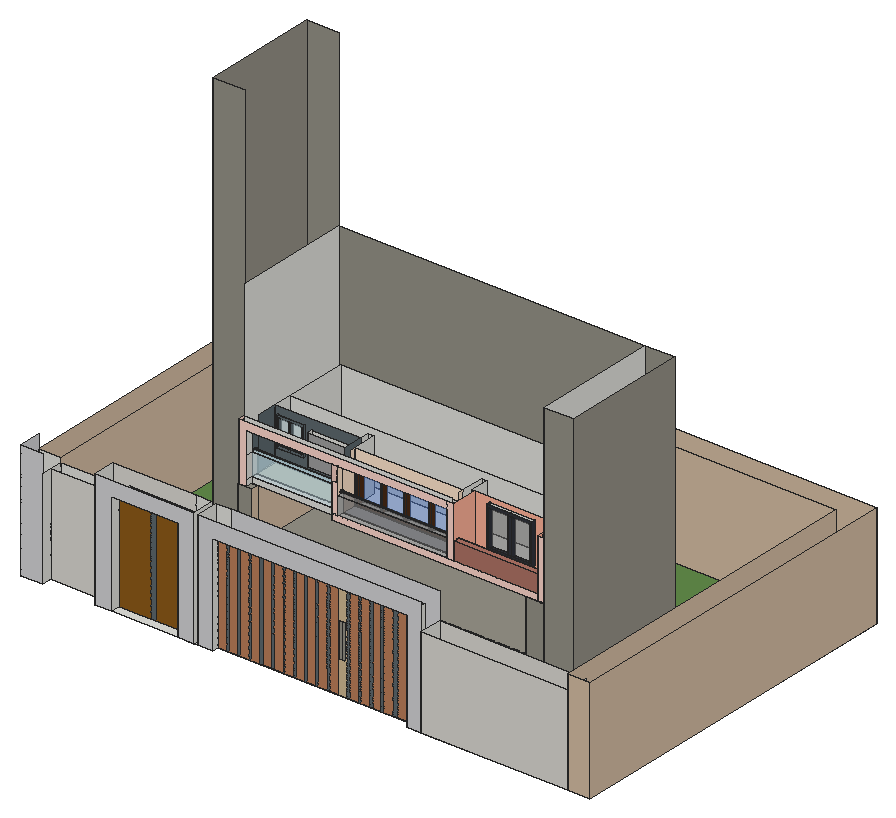
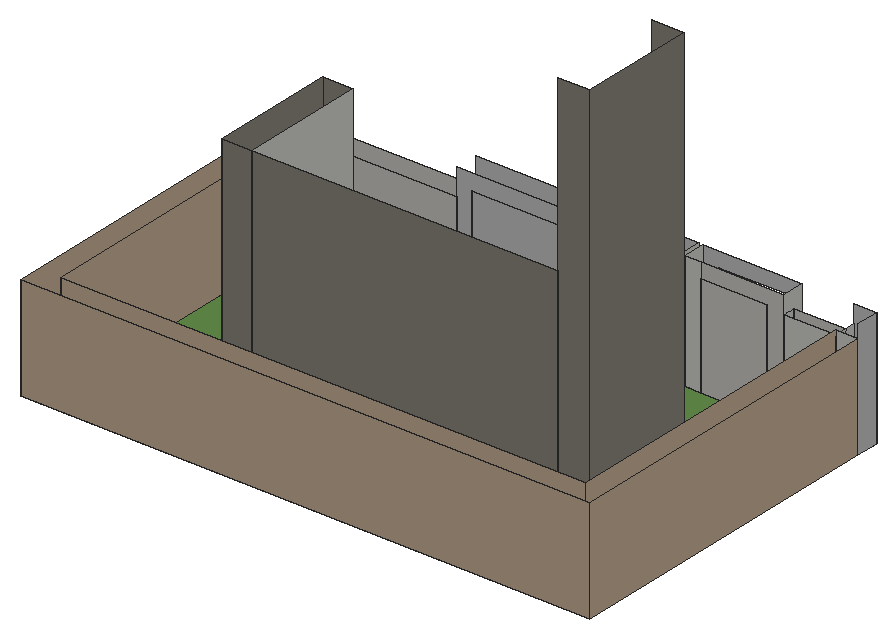
# SketchUp Ruby script. Lengths in inches.
U = 1.inch
M = Sketchup.active_model
def pt(a) = Geom::Point3d.new(a.map { |v| v * U })
def face(e, loops, mat)
  f = e.add_face(loops[0].map { |a| pt(a) })
  loops[1..].each { |l| e.add_face(l.map { |a| pt(a) }).erase! }
  f.material = f.back_material = mat if mat
  f
end
# faces: each face lists its corners as indices into pts; further lists are holes
def faces(e, pts, list, mat = nil) = list.each { |f| face(e, (f[0].is_a?(Array) ? f : [f]).map { |l| l.map { |i| pts[i] } }, mat) }
# xy, xz, yz: faces in a plane at the given z, y or x. An outline is a flat list of corners, or four numbers for a rectangle; further outlines are holes
def ring(l) = l.size == 4 ? [[l[0], l[1]], [l[2], l[1]], [l[2], l[3]], [l[0], l[3]]] : l.each_slice(2).to_a
def flat(e, list, mat, &to3) = list.each { |f| face(e, (f[0].is_a?(Array) ? f : [f]).map { |l| ring(l).map { |u, v| to3.(u, v) } }, mat) }
def xy(e, z, list, mat = nil) = flat(e, list, mat) { |x, y| [x, y, z] }
def xz(e, y, list, mat = nil) = flat(e, list, mat) { |x, z| [x, y, z] }
def yz(e, x, list, mat = nil) = flat(e, list, mat) { |y, z| [x, y, z] }
def lines(e, pts, list) = list.each { |a, b| e.add_line(pt(pts[a]), pt(pts[b])) }
# prism: a flat outline (further loops are holes) pulled along v
def prism(e, loops, v, mat = nil)
  f = face(e, loops, mat); d = Geom::Vector3d.new(v.map { |x| x * U })
  f.pushpull(f.normal.samedirection?(d) ? d.length : -d.length)
end
def box(e, o, s, mat = nil) = prism(e, [[o, [o[0] + s[0], o[1], o[2]], [o[0] + s[0], o[1] + s[1], o[2]], [o[0], o[1] + s[1], o[2]]]], [0, 0, s[2]], mat)
def at(x, y, z, deg = 0) = Geom::Transformation.translation(pt([x, y, z])) * Geom::Transformation.rotation(ORIGIN, Z_AXIS, deg.degrees)
def axes(o, x, y, z) = Geom::Transformation.new([*x, 0, *y, 0, *z, 0, *pt(o).to_a, 1])
def part(name) = M.definitions.add(name)
# library, detail: a bought-in or finely detailed component or shape, given as its bounding box
def library(name, o, s) = part(name).tap { |d| box(d.entities, o, s) }
def detail(e, o, s) = box(e.add_group.entities, o, s)
def put(e, d, t, mat = nil) = e.add_instance(d, t).tap { |i| i.material = mat if mat }
def group(e, t, mat = nil) = e.add_group.tap { |g| g.transformation = t; g.material = mat if mat }.entities
root = M.entities
M.materials.add("[Blinds Vertical Pattern]").color = [212, 212, 214]
M.materials.add("[Blinds Vertical Stripe Gray]").color = [160, 160, 160]
M.materials.add("[Blinds Weave]1").color = [141, 91, 25]
M.materials.add("[Color B01]").color = [255, 216, 204]
M.materials.add("[Color B02]").color = [255, 178, 153]
M.materials.add("[Color C01]").color = [255, 229, 204]
M.materials.add("[Field Rectangle Tile]").color = [196, 189, 179]
M.materials.add("[Field Square Tile]").color = [217, 201, 169]
M.materials.add("[Formica Beige]").color = [211, 187, 149]
M.materials.add("[Formica Graystone]").color = [149, 146, 135]
M.materials.add("[Formica Laminate Dark]").color = [50, 53, 60]
M.materials.add("[Formica Laminate Light]").color = [213, 189, 164]
M.materials.add("[Formica Speckled Grey]").color = [94, 105, 111]
M.materials.add("[Marble Carrara Floor Tile]").color = [204, 208, 219]
M.materials.add("[Stone Flagstone Ashlar]").color = [175, 116, 102]
M.materials.add("[Terrazzo Tile Light]").color = [219, 217, 210]
M.materials.add("[Translucent Glass Blue]").color = [100, 149, 237]
M.materials["[Translucent Glass Blue]"].alpha = 0.5
M.materials.add("[Translucent Glass Gray]").color = [128, 128, 128]
M.materials["[Translucent Glass Gray]"].alpha = 0.5
M.materials.add("[Translucent Glass Safety]").color = [204, 235, 244]
M.materials["[Translucent Glass Safety]"].alpha = 0.5
M.materials.add("[Vegetation Grass Artificial]").color = [98, 140, 74]
M.materials.add("[Wood Veneer 01]").color = [76, 44, 23]
M.materials.add("[Wood Veneer 02]").color = [190, 128, 91]
xy(root,0,[[0,0,137.64,137.64],[3329.24,0,3329.24,2040.55,137.64,2040.55,137.64,137.64,0,137.64,0,2178.1875,3466.875,2178.1875,3466.875,0],[453.55,0,554.87,137.64],[554.87,0,956.3,58.3125],[956.3,0,1057.62,137.64],
  [1057.62,0,1080.95,137.64],[1080.95,0,1170.21,137.64],[2349.69,0,2439.95,137.64],[2439.95,0,3329.24,137.64],[1170.21,42.1875,2349.69,137.64],
  [137.64,62.625,453.55,137.64],[646.49,849.89,2688.89,1616.29],[449.56,899.87,646.49,1616.29]])
xy(root,0,[[[137.64,137.64,3329.24,2040.55],[646.49,849.89,2688.89,849.89,2688.89,1616.29,449.56,1616.29,449.56,899.87,646.49,899.87]]],"[Vegetation Grass Artificial]")
xy(root,9,[[2507.95,849.3125,2688.89,849.89],[2507.95,849.89,2688.89,894.5],[646.49,894.5,646.49,1616.29,2507.95,1616.29,2507.95,894.5,2463.34,894.5,2463.34,1571.68,691.11,1571.68,691.11,894.5],[2507.95,894.5,2688.89,1616.29]])
xy(root,9,[[729.27,849.89,2395.74,894.5],[691.11,894.5,2463.34,1571.68]],"[Formica Graystone]")
xy(root,352.875,[[2395.74,849.89,2507.95,856.3125],[646.49,856.3125,691.11,894.5],[1213.16,856.3125,2395.74,894.5],[2395.74,856.3125,2463.34,894.5],[691.11,894.5,2463.34,1571.68]])
xy(root,352.875,[[646.49,849.89,729.27,849.89,729.27,894.5,691.11,894.5,691.11,856.3125,646.49,856.3125]],"[Formica Graystone]")
xy(root,388.875,[[1213.16,856.3125,1248.61,894.5],[1248.61,856.3125,1908.08,894.5],[1908.08,856.3125,1953.74,894.5],[1953.74,856.3125,2463.34,894.5],[691.11,894.5,1213.16,932.64],
  [1213.16,894.5,1248.61,1126.61],[1908.08,894.5,1908.08,1126.61,1938.3,1126.61,1938.3,1012.29,1953.74,1012.29,1953.74,894.5],[691.11,1182.72,2463.34,1571.68]])
xy(root,388.875,[[1953.74,894.5,2463.34,1012.29]],"[Field Rectangle Tile]")
xy(root,388.875,[[691.11,932.64,1213.16,1074.11]],"[Field Square Tile]")
xy(root,388.875,[[1248.61,894.5,1908.08,983.36]],"[Marble Carrara Floor Tile]")
xy(root,410.6875,[[1285,955.61,1877.875,983.36]])
xy(root,422.97,[[2046.36,990.79,2321.48,1012.29]])
xy(root,427.77,[[1302.08,955.61,1426.75,983.36],[1442.97,955.61,1568.8125,983.36],[1585.03,955.61,1721.6875,983.36],[1737.9,955.61,1860.8,983.36]])
xy(root,436.26,[[2059.65,990.79,2174.84,1012.29],[2197.86,990.79,2308.19,1012.29]],"[Formica Laminate Dark]")
xy(root,458.77,[[914.91,1040.67,1175.1,1074.11]])
xy(root,480.62,[[710.28,1062.73,874.22,1074.11]])
xy(root,493.6,[[723.26,1062.73,783.24,1074.11],[797.04,1062.73,861.24,1074.11]],"[Formica Speckled Grey]")
xy(root,498.24,[[1953.74,856.3125,2463.34,894.5]],"[Stone Flagstone Ashlar]")
xy(root,498.24,[[1248.61,856.3125,1908.08,894.5]],"[Translucent Glass Gray]")
xy(root,523.12,[[691.11,894.5,1213.16,932.64]],"[Translucent Glass Safety]")
xz(root,0,[[0,0,137.64,712.1875],[453.55,0,554.87,0,554.87,623.51,956.3,623.51,956.3,0,1057.62,0,1057.62,712.1875,453.55,712.1875],[1080.95,0,1170.21,0,1170.21,610.51,2349.69,610.51,2349.69,0,2439.95,0,2439.95,712.1875,1080.95,712.1875]],"[Blinds Vertical Pattern]")
xz(root,0,[[3329.24,0,3466.875,631.3125]],"[Formica Laminate Light]")
xz(root,0,[[2439.95,0,3329.24,546.8125]],"[Terrazzo Tile Light]")
xz(root,42.1875,[[[1902.01,0,1953.3,610.51],[1909.36,199.34,1921.17,404.9],[1931.23,199.34,1943.04,404.9]]],"[Formica Beige]")
xz(root,42.1875,[[1909.36,199.34,1921.17,404.9],[1931.23,199.34,1943.04,404.9]],"[Formica Graystone]")
xz(root,42.1875,[[1224.62,0,1235.27,610.51],[1289.68,0,1303.33,610.51],[1357.75,0,1371.39,610.51],[1425.81,0,1439.46,610.51],[1493.87,0,1507.52,610.51],
  [1561.93,0,1575.58,610.51],[1630,0,1643.64,610.51],[1698.06,0,1711.71,610.51],[1766.12,0,1779.65,610.51],[1834.0625,0,1847.59,610.51],
  [1953.3,0,1970.36,610.51],[2024.78,0,2040.05,610.51],[2094.46,0,2108.61,610.51],[2163.03,0,2181.43,610.51],[2235.84,0,2261.55,610.51],
  [2315.96,0,2349.69,610.51]],"[Formica Speckled Grey]")
xz(root,42.1875,[[1170.21,0,1224.62,610.51],[1235.27,0,1289.68,610.51],[1303.33,0,1357.75,610.51],[1371.39,0,1425.81,610.51],[1439.46,0,1493.87,610.51],
  [1507.52,0,1561.93,610.51],[1575.58,0,1630,610.51],[1643.64,0,1698.06,610.51],[1711.71,0,1766.12,610.51],[1779.65,0,1834.0625,610.51],
  [1847.59,0,1902.01,610.51],[1970.36,0,2024.78,610.51],[2040.05,0,2094.46,610.51],[2108.61,0,2163.03,610.51],[2181.43,0,2235.84,610.51],
  [2261.55,0,2315.96,610.51]],"[Wood Veneer 02]")
xz(root,58.3125,[[554.87,0,744.8125,623.51],[776.61,0,956.3,623.51]],"[Blinds Weave]1")
xz(root,58.3125,[[744.8125,0,776.61,623.51]],"[Formica Speckled Grey]")
xz(root,62.625,[[137.64,0,453.55,604.375]],"[Terrazzo Tile Light]")
xz(root,137.64,[[0,0,137.64,631.3125],[137.64,0,453.55,604.375],[956.3,0,1057.62,712.1875],[1080.95,0,1170.21,712.1875]])
xz(root,137.64,[[1170.21,0,2349.69,610.51],[2349.69,0,2349.69,610.51,1170.21,610.51,1170.21,712.1875,2439.95,712.1875,2439.95,0]],"[Blinds Vertical Pattern]")
xz(root,137.64,[[453.55,0,453.55,712.1875,956.3,712.1875,956.3,623.51,554.87,623.51,554.87,0],[554.87,0,956.3,623.51],[2439.95,0,3329.24,546.8125]],"[Terrazzo Tile Light]")
xz(root,849.3125,[[2507.95,9,2688.89,1424.1875]],"[Formica Graystone]")
xz(root,849.89,[[646.49,0,2688.89,0,2688.89,9,2507.95,9,2507.95,352.875,2395.74,352.875,2395.74,9,729.27,9,729.27,352.875,646.49,352.875]],"[Formica Graystone]")
xz(root,856.3125,[[646.49,352.875,691.11,352.875,691.11,657.36,1908.08,657.36,1908.08,702.75,646.49,702.75],[1213.16,352.875,2463.34,388.875],[2463.34,352.875,2507.95,702.75],[1213.16,388.875,1248.61,566.24],[1908.08,388.875,1953.74,702.75]],"[Color B01]")
xz(root,856.3125,[[1953.74,388.875,2463.34,498.24]],"[Stone Flagstone Ashlar]")
xz(root,856.3125,[[1248.61,388.875,1908.08,498.24]],"[Translucent Glass Gray]")
xz(root,894.5,[[646.49,9,691.11,352.875],[691.11,9,729.27,352.875],[2395.74,9,2463.34,352.875],[2463.34,9,2507.95,702.75],[646.49,352.875,646.49,702.75,1908.08,702.75,1908.08,657.36,691.11,657.36,691.11,352.875],
  [691.11,352.875,1213.16,388.875],[1213.16,352.875,2463.34,388.875],[1213.16,388.875,1248.61,657.36],[1953.74,388.875,2463.34,498.24]])
xz(root,894.5,[[1248.61,388.875,1908.08,498.24]],"[Translucent Glass Gray]")
xz(root,894.5,[[691.11,388.875,1213.16,523.12]],"[Translucent Glass Safety]")
xz(root,899.87,[[449.56,0,646.49,2476.875]],"[Formica Graystone]")
xz(root,932.64,[[691.11,388.875,1213.16,523.12]],"[Translucent Glass Safety]")
xz(root,955.61,[[[1285,410.6875,1877.875,636.3125],[1302.08,427.77,1860.8,619.23]],[1426.75,427.77,1442.97,619.23],[1568.8125,427.77,1585.03,619.23],[1721.6875,427.77,1737.9,619.23]],"[Wood Veneer 01]")
xz(root,983.36,[[[1248.61,388.875,1908.08,702.75],[1285,410.6875,1877.875,636.3125]]],"[Color C01]")
xz(root,983.36,[[1302.08,427.77,1426.75,619.23],[1442.97,427.77,1568.8125,619.23],[1585.03,427.77,1721.6875,619.23],[1737.9,427.77,1860.8,619.23]],"[Translucent Glass Blue]")
xz(root,990.79,[[[2046.36,422.97,2321.48,672.85],[2059.65,436.26,2308.19,659.56]],[2174.84,436.26,2197.86,659.56]],"[Formica Laminate Dark]")
xz(root,1012.29,[[1938.3,388.875,1953.74,702.75]])
xz(root,1012.29,[[[1953.74,388.875,2463.34,702.75],[2046.36,422.97,2321.48,672.85]]],"[Color B02]")
xz(root,1012.29,[[2059.65,436.26,2174.84,659.56],[2197.86,436.26,2308.19,659.56]],"[Translucent Glass Gray]")
xz(root,1040.67,[[914.91,458.77,1175.1,642.77]],"[Blinds Vertical Stripe Gray]")
xz(root,1062.73,[[[710.28,480.62,874.22,659.05],[723.26,493.6,861.24,646.07]],[783.24,493.6,797.04,646.07]],"[Formica Speckled Grey]")
xz(root,1074.11,[[[691.11,388.875,1213.16,702.75],[914.91,458.77,1175.1,642.77],[710.28,480.62,874.22,659.05]]],"[Formica Speckled Grey]")
xz(root,1074.11,[[723.26,493.6,783.24,646.07],[797.04,493.6,861.24,646.07]],"[Translucent Glass Safety]")
xz(root,1126.61,[[1213.16,388.875,1248.61,702.75],[1908.08,388.875,1938.3,702.75]])
xz(root,1182.72,[[691.11,388.875,2463.34,702.75]])
xz(root,1571.68,[[691.11,352.875,2463.34,388.875],[691.11,388.875,2463.34,702.75]])
xz(root,1571.68,[[691.11,9,2463.34,352.875]],"[Formica Laminate Light]")
xz(root,1616.29,[[646.49,0,2688.89,9]])
xz(root,1616.29,[[449.56,0,646.49,2476.875],[646.49,9,2507.95,1424.1875],[2507.95,9,2688.89,1424.1875]],"[Formica Graystone]")
xz(root,2040.55,[[137.64,0,3329.24,631.3125]],"[Formica Laminate Light]")
xz(root,2178.1875,[[0,0,3466.875,631.3125]],"[Formica Laminate Light]")
yz(root,0,[[0,0,137.64,712.1875]],"[Blinds Vertical Pattern]")
yz(root,0,[[137.64,0,2178.1875,631.3125]],"[Formica Laminate Light]")
yz(root,137.64,[[0,0,62.625,604.375],[62.625,0,137.64,604.375]])
yz(root,137.64,[[137.64,0,2040.55,631.3125]],"[Formica Laminate Light]")
yz(root,449.56,[[899.87,0,1616.29,2476.875]],"[Formica Graystone]")
yz(root,453.55,[[0,0,0,712.1875,137.64,712.1875,137.64,604.375,62.625,604.375,62.625,0],[62.625,0,137.64,604.375]])
yz(root,554.87,[[0,0,58.3125,623.51],[58.3125,0,137.64,623.51]])
yz(root,646.49,[[849.89,0,849.89,352.875,894.5,352.875,894.5,9,899.87,9,899.87,0],[899.87,0,1616.29,9],[894.5,9,899.87,702.75],[899.87,9,1616.29,1424.1875]])
yz(root,646.49,[[856.3125,352.875,894.5,702.75]],"[Color B01]")
yz(root,691.11,[[856.3125,352.875,894.5,388.875],[894.5,352.875,1571.68,352.875,1571.68,388.875,1182.72,388.875,1182.72,702.75,1074.11,702.75,1074.11,388.875,894.5,388.875],[856.3125,388.875,894.5,523.12],[894.5,388.875,932.64,523.12],[1182.72,388.875,1571.68,702.75],
  [856.3125,523.12,894.5,657.36]])
yz(root,691.11,[[894.5,9,1571.68,352.875]],"[Formica Laminate Light]")
yz(root,691.11,[[[932.64,388.875,950.43,388.875,950.43,657.36,894.5,657.36,894.5,523.12,932.64,523.12],[913.57,529.32,912.64,529.4375,911.77,529.8,911.02,530.37,910.45,531.12,910.09,531.98,909.97,532.92,910.09,533.85,910.45,534.72,911.02,535.46,911.77,536.03,912.64,536.39,913.57,536.52,914.5,536.39,915.37,536.03,916.11,535.46,916.6875,534.72,917.05,533.85,917.17,532.92,917.05,531.98,916.6875,531.12,916.11,530.37,915.37,529.8,914.5,529.4375]],[950.43,388.875,1074.11,702.75]],"[Formica Speckled Grey]")
yz(root,710.28,[[1062.73,480.62,1074.11,659.05]],"[Formica Speckled Grey]")
yz(root,723.26,[[1062.73,493.6,1074.11,646.07]],"[Formica Speckled Grey]")
yz(root,729.27,[[849.89,9,894.5,352.875]],"[Formica Laminate Light]")
yz(root,783.24,[[1062.73,493.6,1074.11,646.07]],"[Formica Speckled Grey]")
yz(root,797.04,[[1062.73,493.6,1074.11,646.07]],"[Formica Speckled Grey]")
yz(root,861.24,[[1062.73,493.6,1074.11,646.07]],"[Formica Speckled Grey]")
yz(root,874.22,[[1062.73,480.62,1074.11,659.05]],"[Formica Speckled Grey]")
yz(root,914.91,[[1040.67,458.77,1074.11,642.77]])
yz(root,956.3,[[0,0,58.3125,623.51],[58.3125,0,137.64,623.51]])
yz(root,1057.62,[[0,0,137.64,712.1875]])
yz(root,1080.95,[[0,0,137.64,712.1875]])
yz(root,1170.21,[[0,0,42.1875,610.51],[42.1875,0,137.64,610.51]])
yz(root,1175.1,[[1040.67,458.77,1074.11,642.77]])
yz(root,1213.16,[[856.3125,352.875,894.5,388.875],[856.3125,388.875,894.5,523.12],[894.5,388.875,932.64,523.12],[1074.11,388.875,1126.61,702.75],[913.57,529.32,914.5,529.4375,915.37,529.8,916.11,530.37,916.6875,531.12,917.05,531.98,917.17,532.92,917.05,533.85,916.6875,534.72,916.11,535.46,915.37,536.03,914.5,536.39,913.57,536.52,912.64,536.39,911.77,536.03,911.02,535.46,910.45,534.72,910.09,533.85,909.97,532.92,910.09,531.98,910.45,531.12,911.02,530.37,911.77,529.8,912.64,529.4375]])
yz(root,1213.16,[[856.3125,523.12,894.5,657.36]],"[Color B01]")
yz(root,1213.16,[[[932.64,388.875,932.64,523.12,894.5,523.12,894.5,657.36,950.43,657.36,950.43,702.75,1074.11,702.75,1074.11,388.875],[913.57,529.32,914.5,529.4375,915.37,529.8,916.11,530.37,916.6875,531.12,917.05,531.98,917.17,532.92,917.05,533.85,916.6875,534.72,916.11,535.46,915.37,536.03,914.5,536.39,913.57,536.52,912.64,536.39,911.77,536.03,911.02,535.46,910.45,534.72,910.09,533.85,909.97,532.92,910.09,531.98,910.45,531.12,911.02,530.37,911.77,529.8,912.64,529.4375]]],"[Formica Speckled Grey]")
yz(root,1248.61,[[856.3125,388.875,894.5,498.24],[983.36,388.875,1126.61,702.75]])
yz(root,1248.61,[[894.5,388.875,983.36,388.875,983.36,702.75,950.43,702.75,950.43,657.36,894.5,657.36],[[856.3125,498.24,894.5,657.36],[876.79,507.06,875.45,507.23,874.2,507.75,873.125,508.58,872.3,509.65,871.78,510.9,871.6,512.24,871.78,513.59,872.3,514.84,873.125,515.91,874.2,516.74,875.45,517.25,876.79,517.43,878.13,517.25,879.39,516.74,880.46,515.91,881.28,514.84,881.8,513.59,881.98,512.24,881.8,510.9,881.28,509.65,880.46,508.58,879.39,507.75,878.13,507.23]]],"[Color C01]")
yz(root,1285,[[955.61,410.6875,983.36,636.3125]],"[Wood Veneer 01]")
yz(root,1302.08,[[955.61,427.77,983.36,619.23]],"[Wood Veneer 01]")
yz(root,1426.75,[[955.61,427.77,983.36,619.23]],"[Wood Veneer 01]")
yz(root,1442.97,[[955.61,427.77,983.36,619.23]],"[Wood Veneer 01]")
yz(root,1568.8125,[[955.61,427.77,983.36,619.23]],"[Wood Veneer 01]")
yz(root,1585.03,[[955.61,427.77,983.36,619.23]],"[Wood Veneer 01]")
yz(root,1721.6875,[[955.61,427.77,983.36,619.23]],"[Wood Veneer 01]")
yz(root,1737.9,[[955.61,427.77,983.36,619.23]],"[Wood Veneer 01]")
yz(root,1860.8,[[955.61,427.77,983.36,619.23]],"[Wood Veneer 01]")
yz(root,1877.875,[[955.61,410.6875,983.36,636.3125]])
yz(root,1908.08,[[856.3125,388.875,894.5,498.24],[983.36,388.875,1126.61,702.75],[876.79,507.06,878.13,507.23,879.39,507.75,880.46,508.58,881.28,509.65,881.8,510.9,881.98,512.24,881.8,513.59,881.28,514.84,880.46,515.91,879.39,516.74,878.13,517.25,876.79,517.43,875.45,517.25,874.2,516.74,873.125,515.91,872.3,514.84,871.78,513.59,871.6,512.24,871.78,510.9,872.3,509.65,873.125,508.58,874.2,507.75,875.45,507.23]])
yz(root,1908.08,[[894.5,388.875,894.5,657.36,950.43,657.36,950.43,702.75,983.36,702.75,983.36,388.875],[[856.3125,498.24,894.5,657.36],[876.79,507.06,878.13,507.23,879.39,507.75,880.46,508.58,881.28,509.65,881.8,510.9,881.98,512.24,881.8,513.59,881.28,514.84,880.46,515.91,879.39,516.74,878.13,517.25,876.79,517.43,875.45,517.25,874.2,516.74,873.125,515.91,872.3,514.84,871.78,513.59,871.6,512.24,871.78,510.9,872.3,509.65,873.125,508.58,874.2,507.75,875.45,507.23]]],"[Color C01]")
yz(root,1938.3,[[1012.29,388.875,1126.61,702.75]])
yz(root,1953.74,[[856.3125,388.875,894.5,498.24]])
yz(root,1953.74,[[[894.5,388.875,1012.29,388.875,1012.29,702.75,856.3125,702.75,856.3125,498.24,894.5,498.24],[876.11,507.08,874.5,507.29,872.99,507.91,871.69,508.91,870.7,510.2,870.08,511.71,869.86,513.33,870.08,514.94,870.7,516.45,871.69,517.75,872.99,518.74,874.5,519.36,876.11,519.58,877.73,519.36,879.24,518.74,880.53,517.75,881.53,516.45,882.15,514.94,882.36,513.33,882.15,511.71,881.53,510.2,880.53,508.91,879.24,507.91,877.73,507.29]]],"[Color B02]")
yz(root,2046.36,[[990.79,422.97,1012.29,672.85]],"[Formica Laminate Dark]")
yz(root,2059.65,[[990.79,436.26,1012.29,659.56]],"[Formica Laminate Dark]")
yz(root,2174.84,[[990.79,436.26,1012.29,659.56]],"[Formica Laminate Dark]")
yz(root,2197.86,[[990.79,436.26,1012.29,659.56]],"[Formica Laminate Dark]")
yz(root,2308.19,[[990.79,436.26,1012.29,659.56]],"[Formica Laminate Dark]")
yz(root,2321.48,[[990.79,422.97,1012.29,672.85]],"[Formica Laminate Dark]")
yz(root,2349.69,[[0,0,42.1875,610.51],[42.1875,0,137.64,610.51]])
yz(root,2395.74,[[849.89,9,894.5,352.875]],"[Formica Graystone]")
yz(root,2439.95,[[0,0,137.64,546.8125]])
yz(root,2463.34,[[856.3125,352.875,894.5,388.875],[894.5,352.875,894.5,388.875,1012.29,388.875,1012.29,702.75,1182.72,702.75,1182.72,388.875,1571.68,388.875,1571.68,352.875],[856.3125,388.875,894.5,498.24],[1182.72,388.875,1571.68,702.75]])
yz(root,2463.34,[[894.5,388.875,1012.29,702.75],[856.3125,498.24,894.5,702.75]],"[Color B02]")
yz(root,2463.34,[[894.5,9,1571.68,352.875]],"[Formica Laminate Light]")
yz(root,2507.95,[[849.3125,9,849.89,702.75],[894.5,9,894.5,702.75,849.3125,702.75,849.3125,1424.1875,1616.29,1424.1875,1616.29,9],[849.89,9,894.5,9,894.5,702.75,856.3125,702.75,856.3125,352.875,849.89,352.875],[849.89,352.875,856.3125,702.75]])
yz(root,2688.89,[[849.89,0,1616.29,9]])
yz(root,2688.89,[[849.3125,9,1616.29,1424.1875]],"[Formica Graystone]")
yz(root,3329.24,[[0,0,137.64,546.8125]])
yz(root,3329.24,[[137.64,0,137.64,546.8125,0,546.8125,0,631.3125,2040.55,631.3125,2040.55,0]],"[Formica Laminate Light]")
yz(root,3466.875,[[0,0,2178.1875,631.3125]],"[Formica Laminate Light]")
p = [[1908.08,876.79,507.06],[1908.08,875.45,507.23],[1248.61,875.45,507.23],[1248.61,876.79,507.06],[1908.08,878.13,507.23],[1248.61,878.13,507.23],
  [1908.08,874.2,507.75],[1248.61,874.2,507.75],[1908.08,879.39,507.75],[1248.61,879.39,507.75],[1908.08,873.125,508.58],[1248.61,873.125,508.58],
  [1908.08,880.46,508.58],[1248.61,880.46,508.58],[1908.08,872.3,509.65],[1248.61,872.3,509.65],[1908.08,881.28,509.65],[1248.61,881.28,509.65],
  [1908.08,871.78,510.9],[1248.61,871.78,510.9],[1908.08,881.8,510.9],[1248.61,881.8,510.9],[1908.08,871.6,512.24],[1248.61,871.6,512.24],
  [1908.08,881.98,512.24],[1248.61,881.98,512.24],[1908.08,871.78,513.59],[1248.61,871.78,513.59],[1908.08,881.8,513.59],[1248.61,881.8,513.59],
  [1908.08,872.3,514.84],[1248.61,872.3,514.84],[1908.08,881.28,514.84],[1248.61,881.28,514.84],[1908.08,873.125,515.91],[1248.61,873.125,515.91],
  [1908.08,880.46,515.91],[1248.61,880.46,515.91],[1908.08,874.2,516.74],[1248.61,874.2,516.74],[1908.08,879.39,516.74],[1248.61,879.39,516.74],
  [1908.08,875.45,517.25],[1248.61,875.45,517.25],[1908.08,878.13,517.25],[1248.61,878.13,517.25],[1908.08,876.79,517.43],[1248.61,876.79,517.43],
  [1213.16,913.57,529.32],[1213.16,912.64,529.4375],[691.11,912.64,529.4375],[691.11,913.57,529.32],[1213.16,914.5,529.4375],[691.11,914.5,529.4375],
  [1213.16,911.77,529.8],[691.11,911.77,529.8],[1213.16,915.37,529.8],[691.11,915.37,529.8],[1213.16,911.02,530.37],[691.11,911.02,530.37],
  [1213.16,916.11,530.37],[691.11,916.11,530.37],[1213.16,910.45,531.12],[691.11,910.45,531.12],[1213.16,916.6875,531.12],[691.11,916.6875,531.12],
  [1213.16,910.09,531.98],[691.11,910.09,531.98],[1213.16,917.05,531.98],[691.11,917.05,531.98],[1213.16,909.97,532.92],[691.11,909.97,532.92],
  [1213.16,917.17,532.92],[691.11,917.17,532.92],[1213.16,910.09,533.85],[691.11,910.09,533.85],[1213.16,917.05,533.85],[691.11,917.05,533.85],
  [1213.16,910.45,534.72],[691.11,910.45,534.72],[1213.16,916.6875,534.72],[691.11,916.6875,534.72],[1213.16,911.02,535.46],[691.11,911.02,535.46],
  [1213.16,916.11,535.46],[691.11,916.11,535.46]]
faces(root,p,[[0,1,2,3],[4,0,3,5],[1,6,7,2],[8,4,5,9],[6,10,11,7],[12,8,9,13],[10,14,15,11],[16,12,13,17],
  [14,18,19,15],[20,16,17,21],[18,22,23,19],[24,20,21,25],[22,26,27,23],[28,24,25,29],[26,30,31,27],[32,28,29,33],
  [30,34,35,31],[36,32,33,37],[34,38,39,35],[40,36,37,41],[38,42,43,39],[44,40,41,45],[42,46,47,43],[46,44,45,47],
  [48,49,50,51],[52,48,51,53],[49,54,55,50],[56,52,53,57],[54,58,59,55],[60,56,57,61],[58,62,63,59],[64,60,61,65],
  [62,66,67,63],[68,64,65,69],[66,70,71,67],[72,68,69,73],[70,74,75,71],[76,72,73,77],[74,78,79,75],[80,76,77,81],
  [78,82,83,79],[84,80,81,85]],"[Formica Laminate Dark]")
